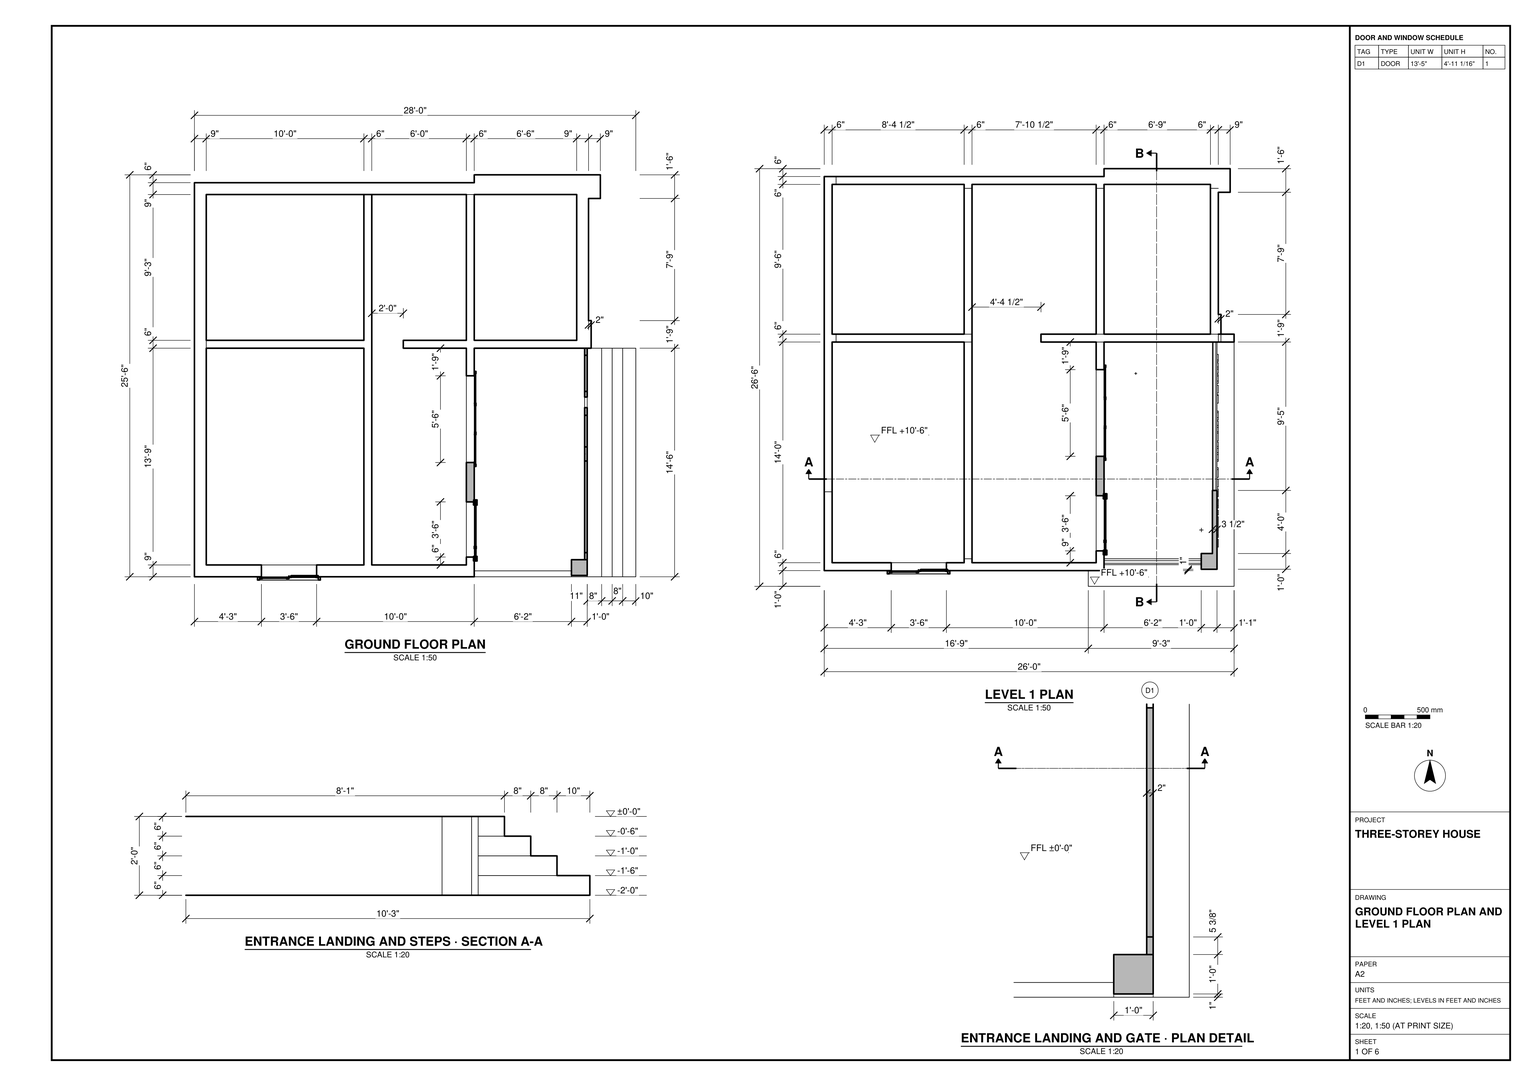
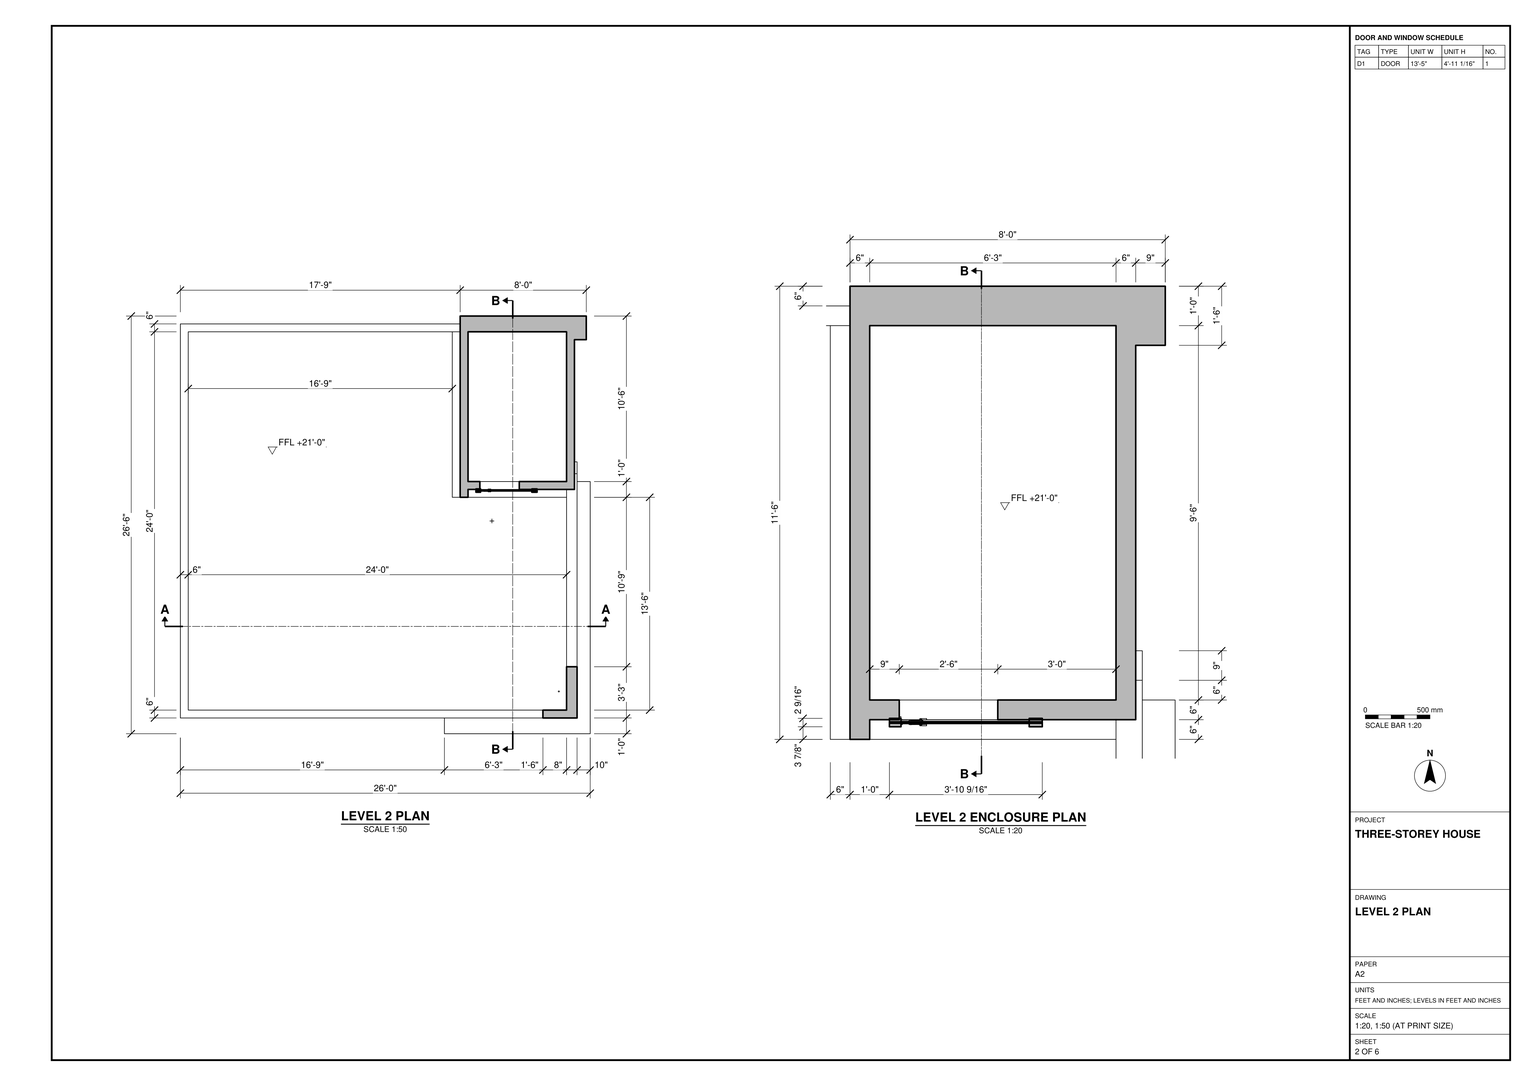
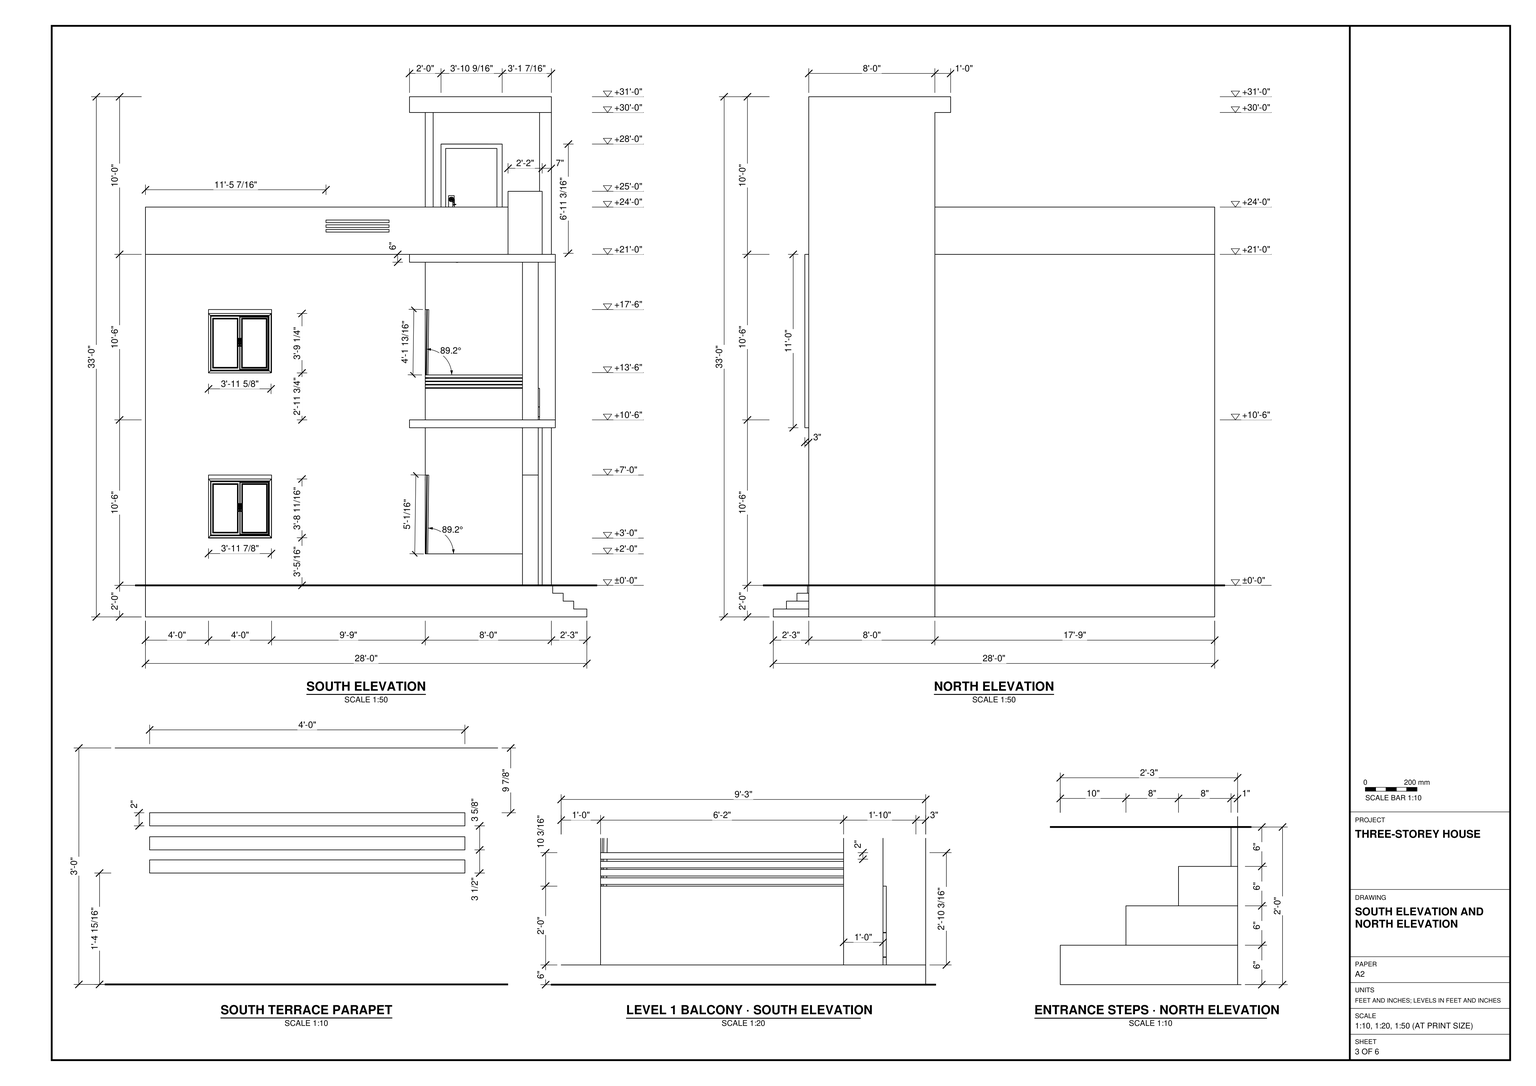
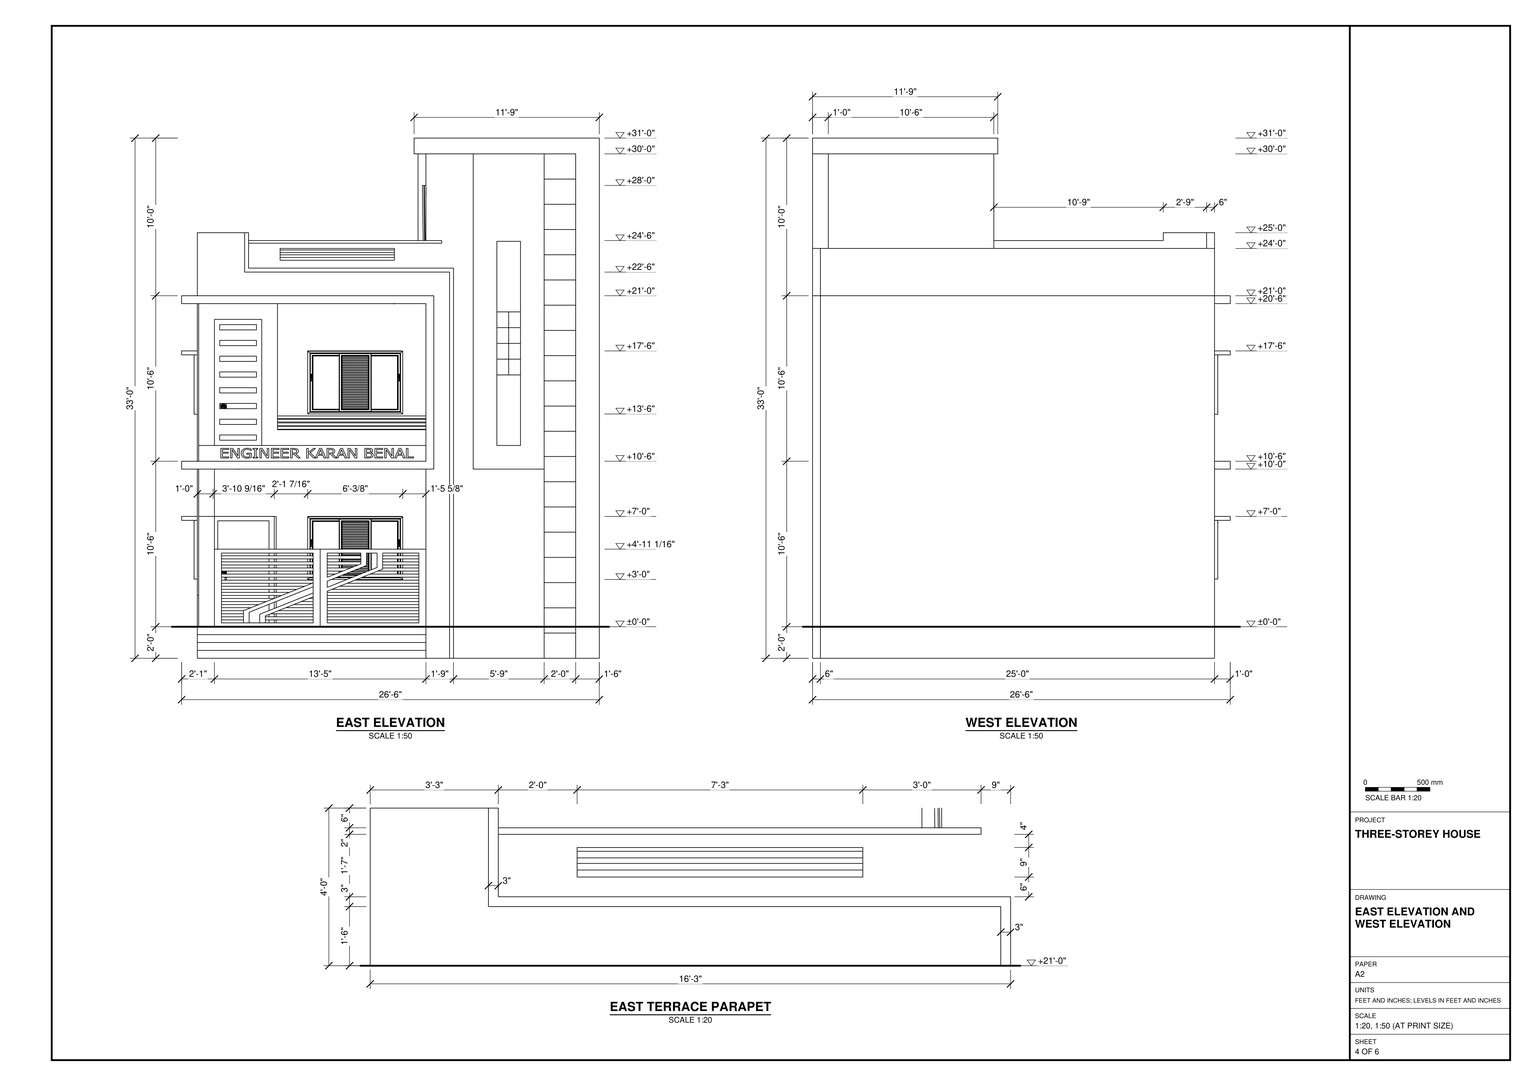
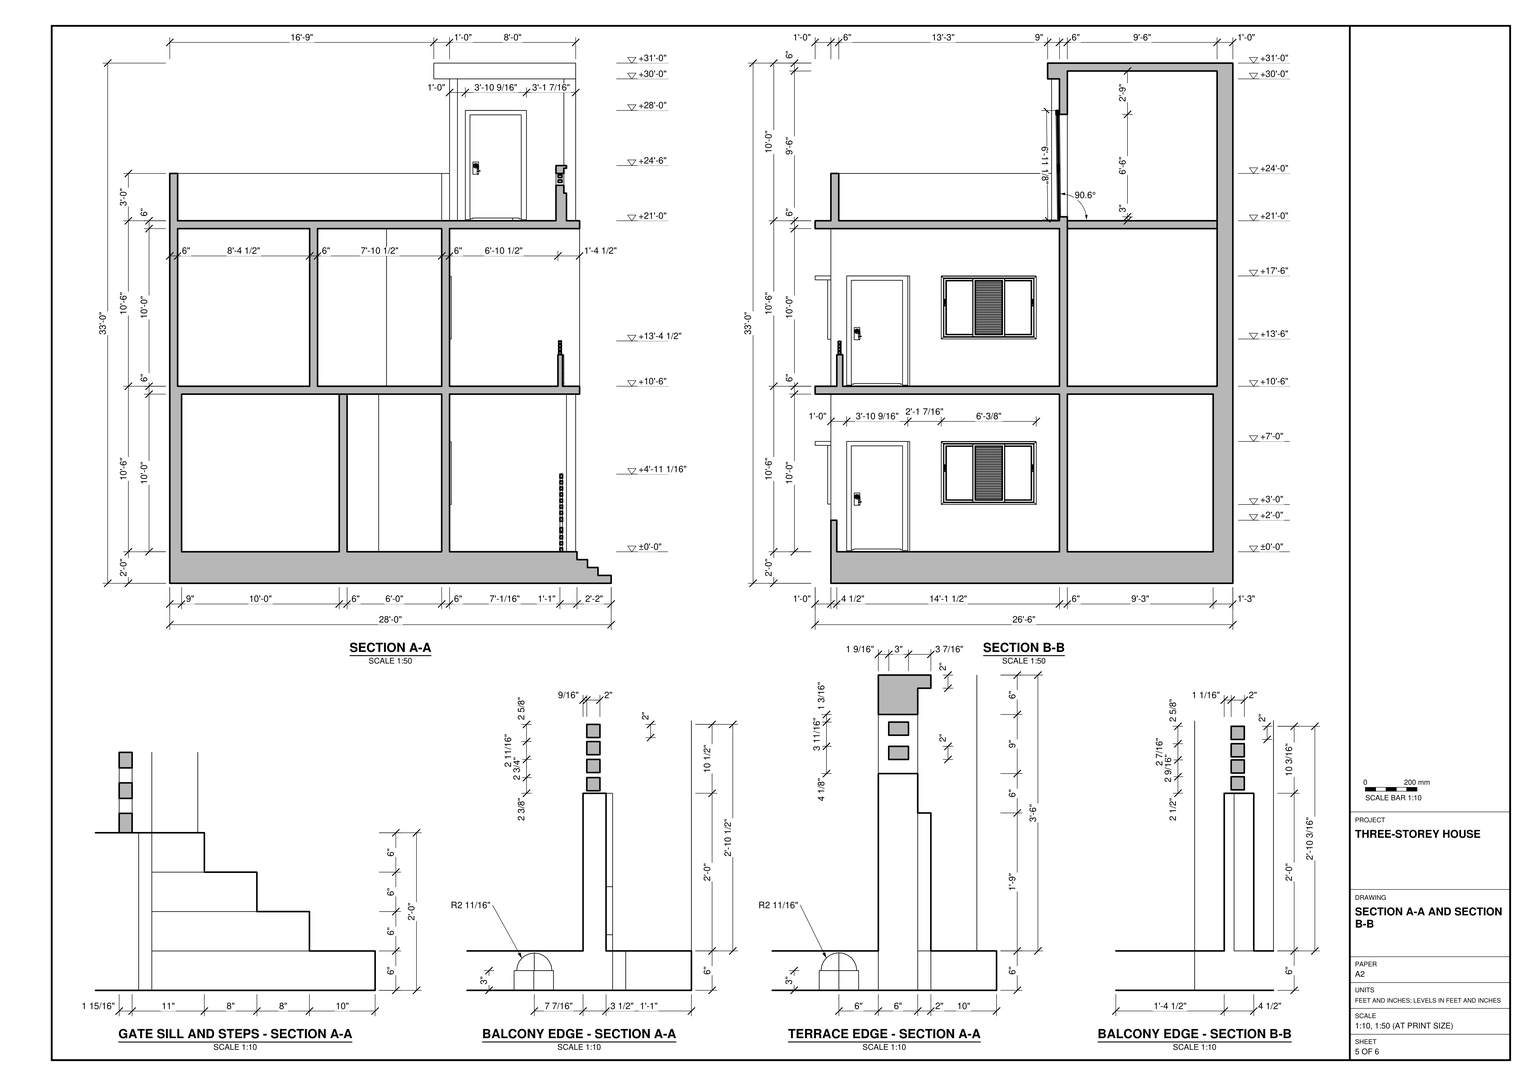
Build the house in SketchUp from task_files/diagram_01.pdf. Work in feet and inches. The overall extents are 28'-0" east to west, 26'-6" north to south and 33'-0" vertically. Set the ground floor at ±0'-0", level 1 at +10'-6" and level 2 at +21'-0". The overall height runs from the base of the entrance steps at -2'-0" to the top of the enclosure roof at +31'-0".

Lay out the lower floors from their respective plans. Follow the wall thicknesses, including the 9" ground-floor perimeter walls and 6" partitions where indicated. Keep the interior openings in their drawn positions rather than copying the ground-floor layout to level 1. Model the entrance landing, steps and gate on the east side, with the projecting balcony slab and horizontal railing above. Align the two south-facing window units as shown in elevation. At level 2, leave the terrace open around the northeast enclosure. Include the terrace parapet, its horizontal detail on the south face, and the enclosure's terrace-facing doorway and projecting flat roof.

Keep walls, slabs, roof elements and any furniture or joinery pieces in separate groups or components, and use components for repeated parts. Decor and loose items, if shown, may be any suitable library components. Save one SketchUp model as output_files/three_storey_house_with_a_balcony_and_roof_terrace.skp.

# SketchUp Ruby script. Lengths in inches.
U = 1.inch
M = Sketchup.active_model
def pt(a) = Geom::Point3d.new(a.map { |v| v * U })
def face(e, loops, mat)
  f = e.add_face(loops[0].map { |a| pt(a) })
  loops[1..].each { |l| e.add_face(l.map { |a| pt(a) }).erase! }
  f.material = f.back_material = mat if mat
  f
end
# faces: each face lists its corners as indices into pts; further lists are holes
def faces(e, pts, list, mat = nil) = list.each { |f| face(e, (f[0].is_a?(Array) ? f : [f]).map { |l| l.map { |i| pts[i] } }, mat) }
# xy, xz, yz: faces in a plane at the given z, y or x. An outline is a flat list of corners, or four numbers for a rectangle; further outlines are holes
def ring(l) = l.size == 4 ? [[l[0], l[1]], [l[2], l[1]], [l[2], l[3]], [l[0], l[3]]] : l.each_slice(2).to_a
def flat(e, list, mat, &to3) = list.each { |f| face(e, (f[0].is_a?(Array) ? f : [f]).map { |l| ring(l).map { |u, v| to3.(u, v) } }, mat) }
def xy(e, z, list, mat = nil) = flat(e, list, mat) { |x, y| [x, y, z] }
def xz(e, y, list, mat = nil) = flat(e, list, mat) { |x, z| [x, y, z] }
def yz(e, x, list, mat = nil) = flat(e, list, mat) { |y, z| [x, y, z] }
def lines(e, pts, list) = list.each { |a, b| e.add_line(pt(pts[a]), pt(pts[b])) }
# prism: a flat outline (further loops are holes) pulled along v
def prism(e, loops, v, mat = nil)
  f = face(e, loops, mat); d = Geom::Vector3d.new(v.map { |x| x * U })
  f.pushpull(f.normal.samedirection?(d) ? d.length : -d.length)
end
def box(e, o, s, mat = nil) = prism(e, [[o, [o[0] + s[0], o[1], o[2]], [o[0] + s[0], o[1] + s[1], o[2]], [o[0], o[1] + s[1], o[2]]]], [0, 0, s[2]], mat)
def at(x, y, z, deg = 0) = Geom::Transformation.translation(pt([x, y, z])) * Geom::Transformation.rotation(ORIGIN, Z_AXIS, deg.degrees)
def axes(o, x, y, z) = Geom::Transformation.new([*x, 0, *y, 0, *z, 0, *pt(o).to_a, 1])
def part(name) = M.definitions.add(name)
# library, detail: a bought-in or finely detailed component or shape, given as its bounding box
def library(name, o, s) = part(name).tap { |d| box(d.entities, o, s) }
def detail(e, o, s) = box(e.add_group.entities, o, s)
def put(e, d, t, mat = nil) = e.add_instance(d, t).tap { |i| i.material = mat if mat }
def group(e, t, mat = nil) = e.add_group.tap { |g| g.transformation = t; g.material = mat if mat }.entities
root = M.entities
M.materials.add("C03_Honey_Glow").color = [255, 178, 101]
M.materials.add("Carpet_04_1K").color = [43, 65, 85]
M.materials.add("D05_Goldenrod_Hue").color = [255, 191, 0]
M.materials.add("[_0053_Ivory_]").color = [200, 200, 200]
c1 = library("porta+4",[0.2,-5.42,1.33],[46.55,4.72,83.21])
c2 = library("Modern+Gate+1",[0,0,0],[118.11,1.97,78.74])
c3 = library("ENGINEER KARAN B",[0.96,0,0],[146.72,9.87,1])
c4 = library("Sphere Light",[-2.72,-2.72,-2.72],[5.44,5.44,5.44])
c5 = library("Sphere Light\#1",[-3.15,-3.15,-3.15],[6.3,6.3,6.3])
c6 = library("Sphere Light\#2",[-2.75,-2.75,-2.75],[5.5,5.5,5.5])
c7 = library("Sphere Light\#3",[-2.83,-2.83,-2.83],[5.66,5.66,5.66])
c8 = library("Sphere Light\#4",[-3.12,-3.12,-3.12],[6.24,6.24,6.24])
c9 = library("Sphere Light\#5",[-2.55,-2.55,-2.55],[5.1,5.1,5.1])
c10 = library("Sphere Light\#6",[-2.68,-2.68,-2.68],[5.36,5.36,5.36])
c11 = library("Sphere Light\#7",[-2.9,-2.9,-2.9],[5.8,5.8,5.8])
c12 = library("mesh-166",[-1553.69,-2604.3125,-42.18],[1702.88,1401.6,88.28])
c13 = part("Group17")
put(c13.entities,c12,at(294.66,859.51,3.5))
c14 = library("mesh-160",[-91.39,-1008.79,-36.9],[2366.42,1739.16,65.81])
c15 = part("Group4")
g1 = group(c15.entities,at(-5.75,-6.15,0))
put(g1,c14,axes([0,0,0],[1,0,0],[0,0,1],[0,-1,0]))
put(root,c1,at(224.8,188.76,275.46))
put(root,c1,at(210.24,23.8,23.48,90))
put(root,c1,at(210.24,23.8,149.48,90))
put(root,c2,axes([299,25,24],[0,1.36313,0],[-1,0,0],[0,0,0.75]))
g2 = group(root,at(0,72,0),"[_0053_Ivory_]")
xy(g2,0,[[0,-60,0,240,213,240,213,246,309,246,309,228,300,228,300,135,302,135,302,114,336,114,336,-60]])
xy(g2,6,[[326,-60,336,114]])
xy(g2,12,[[318,-60,326,114]])
xy(g2,18,[[310,-60,318,114]])
xy(g2,24,[[287,-60,299,-59],[299,-60,310,114],[213,-55.5,287,-55.5,287,-47,299,-47,299,114,213,114],[9,-51,129,114],[135,-51,207,-51,207,114,159,114,159,120,207,120,207,231,135,231],
  [9,120,129,231],[213,120,291,231]])
xy(g2,27,[[207,-45,213,-3]])
xy(g2,48,[[213,-60,287,-55.5]])
xy(g2,63,[[51,-60,93,-51],[207,27,213,93]])
xy(g2,105,[[48,-72,48,-60,51,-60,51,-51,93,-51,93,-60,96,-60,96,-72],[207,-45,213,-3],[207,27,213,93]])
xy(g2,108,[[48,-72,96,-60],[287,-59,299,-47]])
xy(g2,144,[[[201,-72,201,-60,213,-60,213,114,302,114,302,120,312,120,312,-72],[287,-59,299,-47],[237,87,237.78,87.1,238.5,87.4,239.12,87.88,239.6,88.5,239.9,89.22,240,90,239.9,90.78,239.6,91.5,239.12,92.12,238.5,92.6,237.78,92.9,237,93,236.22,92.9,235.5,92.6,234.88,92.12,234.4,91.5,234.1,90.78,234,90,234.1,89.22,234.4,88.5,234.88,87.88,235.5,87.4,236.22,87.1],[288,87,288.78,87.1,289.5,87.4,290.12,87.88,290.6,88.5,290.9,89.22,291,90,290.9,90.78,290.6,91.5,290.12,92.12,289.5,92.6,288.78,92.9,288,93,287.22,92.9,286.5,92.6,285.88,92.12,285.4,91.5,285.1,90.78,285,90,285.1,89.22,285.4,88.5,285.88,87.88,286.5,87.4,287.22,87.1],[237,-31.89,237.78,-31.79,238.5,-31.49,239.12,-31.01,239.6,-30.39,239.9,-29.66,240,-28.89,239.9,-28.11,239.6,-27.39,239.12,-26.77,238.5,-26.29,237.78,-25.99,237,-25.89,236.22,-25.99,235.5,-26.29,234.88,-26.77,234.4,-27.39,234.1,-28.11,234,-28.89,234.1,-29.66,234.4,-30.39,234.88,-31.01,235.5,-31.49,236.22,-31.79],[287.25,-31.88,288,-31.71,288.01,-31.71,288.71,-31.35,289.29,-30.83,289.71,-30.17,289.95,-29.42,289.99,-28.64,289.82,-27.875,289.47,-27.18,288.94,-26.6,288.28,-26.18,288,-26.08,287.54,-25.9375,286.75,-25.9,285.99,-26.0625,285.29,-26.42,284.71,-26.95,284.29,-27.61,284.05,-28.35,284.02,-28.89,284.01,-29.13,284.18,-29.9,284.53,-30.6,285.06,-31.18,285.72,-31.6,286.46,-31.84]],[287,-59,287,-48,288,-48,288,-47,299,-47,299,-59],[129,-51,135,-51,135,120,9,120,9,114,129,114],[9,-51,129,114],[135,-51,207,114],
  [287,-48,288,-47],[135,114,159,120],[9,120,129,231],[129,120,135,231],[135,120,207,231],
  [207,120,213,231],[213,120,291,231]])
xy(g2,147,[[237,-31.89,236.22,-31.79,235.5,-31.49,234.88,-31.01,234.4,-30.39,234.1,-29.66,234,-28.89,234.1,-28.11,234.4,-27.39,234.88,-26.77,235.5,-26.29,236.22,-25.99,237,-25.89,237.78,-25.99,238.5,-26.29,239.12,-26.77,239.6,-27.39,239.9,-28.11,240,-28.89,239.9,-29.66,239.6,-30.39,239.12,-31.01,238.5,-31.49,237.78,-31.79],[287.25,-31.88,286.46,-31.84,285.72,-31.6,285.06,-31.18,284.53,-30.6,284.18,-29.9,284.01,-29.13,284.02,-28.89,284.05,-28.35,284.29,-27.61,284.71,-26.95,285.29,-26.42,285.99,-26.0625,286.75,-25.9,287.54,-25.9375,288,-26.08,288.28,-26.18,288.94,-26.6,289.47,-27.18,289.82,-27.875,289.99,-28.64,289.95,-29.42,289.71,-30.17,289.29,-30.83,288.71,-31.35,288.01,-31.71,288,-31.71],[237,87,236.22,87.1,235.5,87.4,234.88,87.88,234.4,88.5,234.1,89.22,234,90,234.1,90.78,234.4,91.5,234.88,92.12,235.5,92.6,236.22,92.9,237,93,237.78,92.9,238.5,92.6,239.12,92.12,239.6,91.5,239.9,90.78,240,90,239.9,89.22,239.6,88.5,239.12,87.88,238.5,87.4,237.78,87.1],[288,87,287.22,87.1,286.5,87.4,285.88,87.88,285.4,88.5,285.1,89.22,285,90,285.1,90.78,285.4,91.5,285.88,92.12,286.5,92.6,287.22,92.9,288,93,288.78,92.9,289.5,92.6,290.12,92.12,290.6,91.5,290.9,90.78,291,90,290.9,89.22,290.6,88.5,290.12,87.88,289.5,87.4,288.78,87.1]])
xy(g2,150,[[201,-72,312,-72,312,114,299,114,299,-59,287,-59,287,-55.5,213,-55.5,213,-60,201,-60],[287,-59,299,-47],[6,-54,106.5,114],[112.5,-54,207,-54,207,114,165,114,165,120,207,120,207,234,112.5,234],[213,-51,287,-51,287,-47,295.5,-47,295.5,114,213,114],
  [6,120,106.5,234],[213,120,294,234]])
xy(g2,153,[[207,-45,213,-3]])
xy(g2,166,[[295.5,-43,299,-15]])
xy(g2,170,[[295.5,-43,299,-15]])
xy(g2,174,[[213,-55.5,287,-51],[295.5,1,299,114]])
xy(g2,174.39,[[296.07,1,298.07,114]])
xy(g2,174.52,[[213,-54.44,287,-52.44]])
xy(g2,176.39,[[296.07,1,298.07,114]])
xy(g2,176.52,[[213,-54.44,287,-52.44]])
xy(g2,177.08,[[213,-54.44,287,-52.44]])
xy(g2,177.16,[[296.07,1,298.07,114]])
xy(g2,178,[[295.5,-43,299,-15]])
xy(g2,179.08,[[213,-54.44,287,-52.44]])
xy(g2,179.16,[[296.07,1,298.07,114]])
xy(g2,179.55,[[213,-54.44,287,-52.44]])
xy(g2,179.875,[[296.07,1,298.07,114]])
xy(g2,181.55,[[213,-54.44,287,-52.44]])
xy(g2,181.875,[[296.07,1,298.07,114]])
xy(g2,182,[[295.5,-43,299,-15]])
xy(g2,182.2,[[213,-54.44,287,-52.44]])
xy(g2,182.49,[[296.07,1,298.07,114]])
xy(g2,184.2,[[213,-54.44,287,-52.44]])
xy(g2,184.49,[[296.07,1,298.07,114]])
xy(g2,189,[[51,-60,93,-54],[207,27,213,93]])
xy(g2,190,[[295.5,-43,299,-15]])
xy(g2,194,[[295.5,-43,299,-15]])
xy(g2,202,[[295.5,-43,299,-15]])
xy(g2,206,[[295.5,-43,299,-15]])
xy(g2,214,[[295.5,-43,299,-15]])
xy(g2,218,[[295.5,-43,299,-15]])
xy(g2,226,[[295.5,-43,299,-15]])
xy(g2,230,[[295.5,-43,299,-15]])
xy(g2,231,[[48,-72,48,-60,51,-60,51,-54,93,-54,93,-60,96,-60,96,-72],[207,-45,213,-3],[207,27,213,93]])
xy(g2,234,[[48,-72,96,-60]])
xy(g2,238,[[295.5,-43,299,-15]])
xy(g2,242,[[295.5,-43,299,-15]])
xy(g2,250,[[295.5,-43,299,-15]])
xy(g2,254,[[295.5,-43,299,-15]])
xy(g2,270,[[[201,-72,201,-60,213,-60,213,114,312,114,312,-72],[287,-59,299,-59,299,1,295.5,1,295.5,-47,287,-47],[237,-42.92,237.78,-42.82,238.5,-42.52,239.12,-42.04,239.6,-41.42,239.9,-40.7,240,-39.92,239.9,-39.14,239.6,-38.42,239.12,-37.8,238.5,-37.32,237.78,-37.02,237,-36.92,236.22,-37.02,235.5,-37.32,234.88,-37.8,234.4,-38.42,234.1,-39.14,234,-39.92,234.1,-40.7,234.4,-41.42,234.88,-42.04,235.5,-42.52,236.22,-42.82],[237,87,237.78,87.1,238.5,87.4,239.12,87.88,239.6,88.5,239.9,89.22,240,90,239.9,90.78,239.6,91.5,239.12,92.12,238.5,92.6,237.78,92.9,237,93,236.22,92.9,235.5,92.6,234.88,92.12,234.4,91.5,234.1,90.78,234,90,234.1,89.22,234.4,88.5,234.88,87.88,235.5,87.4,236.22,87.1],[288,87,288.78,87.1,289.5,87.4,290.12,87.88,290.6,88.5,290.9,89.22,291,90,290.9,90.78,290.6,91.5,290.12,92.12,289.5,92.6,288.78,92.9,288,93,287.22,92.9,286.5,92.6,285.88,92.12,285.4,91.5,285.1,90.78,285,90,285.1,89.22,285.4,88.5,285.88,87.88,286.5,87.4,287.22,87.1],[288,-42.92,288.78,-42.82,289.5,-42.52,290.12,-42.04,290.6,-41.42,290.9,-40.7,291,-39.92,290.9,-39.14,290.6,-38.42,290.12,-37.8,289.5,-37.32,288.78,-37.02,288,-36.92,287.22,-37.02,286.5,-37.32,285.88,-37.8,285.4,-38.42,285.1,-39.14,285,-39.92,285.1,-40.7,285.4,-41.42,285.88,-42.04,286.5,-42.52,287.22,-42.82]],[287,-59,287,-48,288,-48,288,-47,295.5,-47,295.5,1,299,1,299,-59],[6,-54,106.5,114],[112.5,-54,165,234],[165,-54,207,114],
  [287,-48,288,-47],[6,114,106.5,120],[165,114,207,120],[6,120,106.5,234],[165,120,207,234],
  [213,120,294,234]])
xy(g2,273,[[237,-42.92,236.22,-42.82,235.5,-42.52,234.88,-42.04,234.4,-41.42,234.1,-40.7,234,-39.92,234.1,-39.14,234.4,-38.42,234.88,-37.8,235.5,-37.32,236.22,-37.02,237,-36.92,237.78,-37.02,238.5,-37.32,239.12,-37.8,239.6,-38.42,239.9,-39.14,240,-39.92,239.9,-40.7,239.6,-41.42,239.12,-42.04,238.5,-42.52,237.78,-42.82],[288,-42.92,287.22,-42.82,286.5,-42.52,285.88,-42.04,285.4,-41.42,285.1,-40.7,285,-39.92,285.1,-39.14,285.4,-38.42,285.88,-37.8,286.5,-37.32,287.22,-37.02,288,-36.92,288.78,-37.02,289.5,-37.32,290.12,-37.8,290.6,-38.42,290.9,-39.14,291,-39.92,290.9,-40.7,290.6,-41.42,290.12,-42.04,289.5,-42.52,288.78,-42.82],[237,87,236.22,87.1,235.5,87.4,234.88,87.88,234.4,88.5,234.1,89.22,234,90,234.1,90.78,234.4,91.5,234.88,92.12,235.5,92.6,236.22,92.9,237,93,237.78,92.9,238.5,92.6,239.12,92.12,239.6,91.5,239.9,90.78,240,90,239.9,89.22,239.6,88.5,239.12,87.88,238.5,87.4,237.78,87.1],[288,87,287.22,87.1,286.5,87.4,285.88,87.88,285.4,88.5,285.1,89.22,285,90,285.1,90.78,285.4,91.5,285.88,92.12,286.5,92.6,287.22,92.9,288,93,288.78,92.9,289.5,92.6,290.12,92.12,290.6,91.5,290.9,90.78,291,90,290.9,89.22,290.6,88.5,290.12,87.88,289.5,87.4,288.78,87.1]])
xy(g2,276,[[201,-72,312,-72,312,120,302,120,302,-60,201,-60],[6,-54,294,-54,294,108,207,108,207,234,6,234],[207,108,213,234],[219,108,294,114],[213,120,219,234],
  [219,120,294,234]])
xy(g2,276,[[300,114,302,120]],"Carpet_04_1K")
xy(g2,279,[[228,114,258,120]])
xy(g2,292.96,[[137.43,-60,185.43,-54]])
xy(g2,294.96,[[137.43,-60,185.43,-54]])
xy(g2,296.49,[[137.43,-60,185.43,-54]])
xy(g2,297,[[300,-21,302,135]])
xy(g2,298.49,[[137.43,-60,185.43,-54]])
xy(g2,300.14,[[137.43,-60,185.43,-54]])
xy(g2,302.14,[[137.43,-60,185.43,-54]])
xy(g2,303,[[294,3,300,90]])
xy(g2,305.15,[[295.59,3,298.59,90]])
xy(g2,307.15,[[295.59,3,298.59,90]])
xy(g2,308.84,[[295.59,3,298.59,90]])
xy(g2,310.84,[[295.59,3,298.59,90]])
xy(g2,312,[[0,-60,276,-60,276,-54,6,-54,6,234,213,234,213,240,0,240],[294,3,300,90]])
xy(g2,316,[[300,-21,302,114],[300,114,302,126]])
xy(g2,318,[[294,-21,302,-21,302,126,300,126,300,114,294,114]])
xy(g2,324,[[276,-60,302,-60,302,-21,294,-21,294,-54,276,-54]])
xy(g2,357,[[228,114,258,120]])
xy(g2,384,[[201,105,201,114,213,114,213,108,219,108,219,114,300,114,300,228,309,228,309,105],[201,114,213,234],[201,234,213,246]])
xy(g2,390,[[219,120,294,234]])
xy(g2,396,[[201,105,309,246]])
xz(g2,-72,[[48,105,96,108],[201,144,312,150],[48,231,96,234],[201,270,312,276]])
xz(g2,-60,[[[0,0,336,0,336,6,326,6,326,12,318,12,318,18,310,18,310,24,287,24,287,48,213,48,213,144,201,144,201,150,213,150,213,270,201,270,201,276,0,276],[48,186,96,234],[48,60,96,108]],[48,60,96,60,96,105,93,105,93,63,51,63,51,105,48,105],[48,186,96,186,96,231,93,231,93,189,51,189,51,231,48,231],[[0,276,276,312],[137.43,300.14,185.43,302.14],[137.43,296.49,185.43,298.49],[137.43,292.96,185.43,294.96]]])
xz(g2,-60,[[276,276,302,324]],"Carpet_04_1K")
xz(g2,-59,[[287,108,299,144],[287,144,299,150],[287,150,299,270]])
xz(g2,-59,[[287,24,299,108]],"Carpet_04_1K")
xz(g2,-55.5,[[213,24,287,48],[213,150,287,174]])
xz(g2,-54.44,[[213,174.52,287,176.52],[213,177.08,287,179.08],[213,179.55,287,181.55],[213,182.2,287,184.2]])
xz(g2,-54,[[[6,150,106.5,270],[51,189,93,231]],[112.5,150,207,270],[[6,276,6,312,276,312,276,324,294,324,294,276],[137.43,292.96,185.43,294.96],[137.43,296.49,185.43,298.49],[137.43,300.14,185.43,302.14]]])
xz(g2,-52.44,[[213,174.52,287,176.52],[213,177.08,287,179.08],[213,179.55,287,181.55],[213,182.2,287,184.2]])
xz(g2,-51,[[[9,24,129,144],[51,63,93,105]],[135,24,207,144],[213,150,287,174]])
xz(g2,-47,[[287,108,299,144],[287,144,299,150],[287,150,295.5,270]])
xz(g2,-47,[[287,24,299,108]],"Carpet_04_1K")
xz(g2,-45,[[207,27,213,105],[207,153,213,231]])
xz(g2,-43,[[295.5,166,299,170],[295.5,178,299,182],[295.5,190,299,194],[295.5,202,299,206],[295.5,214,299,218],
  [295.5,226,299,230],[295.5,238,299,242],[295.5,250,299,254]])
xz(g2,-31.71,[[288,144,288.01,147]])
xz(g2,-21,[[300,297,302,316],[294,318,302,324]])
xz(g2,-15,[[295.5,166,299,170],[295.5,178,299,182],[295.5,190,299,194],[295.5,202,299,206],[295.5,214,299,218],
  [295.5,226,299,230],[295.5,238,299,242],[295.5,250,299,254]])
xz(g2,-3,[[207,27,213,105],[207,153,213,231]])
xz(g2,1,[[[295.5,174,299,270],[296.07,174.39,298.07,176.39],[296.07,177.16,298.07,179.16],[296.07,179.875,298.07,181.875],[296.07,182.49,298.07,184.49]]])
xz(g2,3,[[[294,303,300,312],[295.59,308.84,298.59,310.84],[295.59,305.15,298.59,307.15]]])
xz(g2,27,[[207,63,213,105],[207,189,213,231]])
xz(g2,90,[[[294,303,300,312],[295.59,308.84,298.59,310.84],[295.59,305.15,298.59,307.15]]])
xz(g2,93,[[207,63,213,105],[207,189,213,231]])
xz(g2,105,[[201,384,309,396]])
xz(g2,108,[[213,276,219,384]])
xz(g2,114,[[302,0,336,6],[302,6,326,12],[302,12,318,18],[302,18,310,24],[9,24,129,144],
  [159,24,207,144],[213,24,302,144],[6,150,106.5,270],[165,150,207,270],[[213,150,295.5,150,295.5,174,300,174,300,150,312,150,312,270,213,270],[296.07,182.49,298.07,184.49],[296.07,179.875,298.07,181.875],[296.07,177.16,298.07,179.16],[296.07,174.39,298.07,176.39]],
  [299,150,300,174],[219,276,225,276,225,360,261,360,261,276,294,276,294,318,300,318,300,384,219,384],[[225,276,261,360],[228,279,258,357]]])
xz(g2,120,[[9,24,129,144],[159,24,207,144],[213,24,291,144],[302,144,312,276],[6,150,106.5,270],
  [165,150,207,270],[213,150,294,270],[213,270,294,276],[[219,276,294,390],[228,279,258,357]]])
xz(g2,120,[[300,150,302,276]],"Carpet_04_1K")
xz(g2,126,[[300,316,302,318]])
xz(g2,135,[[300,0,302,297]])
xz(g2,228,[[300,0,309,384]])
xz(g2,231,[[9,24,129,144],[129,24,135,144],[135,24,207,144],[213,24,291,144]])
xz(g2,234,[[6,150,106.5,270],[112.5,150,207,270],[213,150,294,270],[213,270,294,276],[6,276,207,312],
  [207,276,213,312],[219,276,294,390]])
xz(g2,240,[[0,0,213,276],[0,276,213,312]])
xz(g2,246,[[213,0,213,384,201,384,201,396,309,396,309,0]])
yz(g2,0,[[-60,0,240,276],[-60,276,240,312]])
yz(g2,6,[[-54,150,114,270],[120,150,234,270],[-54,276,234,312]])
yz(g2,9,[[-51,24,114,144],[120,24,231,144]])
yz(g2,48,[[-72,105,-60,108],[-72,231,-60,234]])
yz(g2,51,[[-60,63,-51,105],[-60,189,-54,231]])
yz(g2,93,[[-60,63,-51,105],[-60,189,-54,231]])
yz(g2,96,[[-72,105,-60,108],[-72,231,-60,234]])
yz(g2,106.5,[[-54,150,114,270],[120,150,234,270]])
yz(g2,112.5,[[-54,150,234,270]])
yz(g2,129,[[-51,24,114,144],[120,24,231,144]])
yz(g2,135,[[-51,24,120,144],[120,24,231,144]])
yz(g2,137.43,[[-60,292.96,-54,294.96],[-60,296.49,-54,298.49],[-60,300.14,-54,302.14]])
yz(g2,159,[[114,24,120,144]])
yz(g2,165,[[114,150,120,270]])
yz(g2,185.43,[[-60,292.96,-54,294.96],[-60,296.49,-54,298.49],[-60,300.14,-54,302.14]])
yz(g2,201,[[-72,144,-60,150],[-72,270,-60,276],[105,384,246,396]])
yz(g2,207,[[[-51,24,114,144],[-45,27,-3,105],[27,63,93,105]],[120,24,231,144],[[-54,150,114,270],[-45,153,-3,231],[27,189,93,231]],[120,150,234,270]])
yz(g2,213,[[240,0,246,276],[[-55.5,24,-48,24,-48,108,0,108,0,24,114,24,114,144,-60,144,-60,48,-55.5,48],[24,60,96,108]],[[-48,24,0,108],[-45,27,-3,105]],[120,24,231,144],[[24,60,96,108],[27,63,93,105]],
  [[-60,150,-55.5,150,-55.5,174,-51,174,-51,150,-48,150,-48,234,0,234,0,150,114,150,114,270,-60,270],[24,186,96,234],[-54.44,174.52,-52.44,176.52],[-54.44,177.08,-52.44,179.08],[-54.44,179.55,-52.44,181.55],[-54.44,182.2,-52.44,184.2]],[[-48,150,0,234],[-45,153,-3,231]],[120,150,234,270],[-54.44,174.52,-52.44,176.52],[-54.44,177.08,-52.44,179.08],
  [-54.44,179.55,-52.44,181.55],[-54.44,182.2,-52.44,184.2],[[24,186,96,234],[27,189,93,231]],[114,270,120,276],[108,276,234,384],
  [240,276,246,312],[234,312,246,384]])
yz(g2,219,[[108,276,114,384],[120,276,234,390]])
yz(g2,228,[[114,279,120,357]])
yz(g2,258,[[114,279,120,357]])
yz(g2,276,[[-60,312,-54,324]])
yz(g2,287,[[-60,24,-59,48],[-59,24,-55.5,48],[-59,108,-47,144],[-59,144,-47,150],[[-59,150,-59,270,-47,270,-47,150,-51,150,-51,174,-55.5,174,-55.5,150],[-54.44,182.2,-52.44,184.2],[-54.44,179.55,-52.44,181.55],[-54.44,177.08,-52.44,179.08],[-54.44,174.52,-52.44,176.52]]])
yz(g2,287,[[-55.5,24,-55.5,48,-59,48,-59,108,-47,108,-47,24]],"Carpet_04_1K")
yz(g2,291,[[120,24,231,144]])
yz(g2,294,[[120,150,234,270],[120,270,234,276],[[-54,276,-54,324,-21,324,-21,318,108,318,108,276],[3,303,90,312]],[108,276,114,318],[120,276,234,390]])
yz(g2,295.5,[[[-47,150,114,174],[-43,166,-15,170]],[[-47,174,1,270],[-43,178,-15,182],[-43,190,-15,194],[-43,202,-15,206],[-43,214,-15,218],[-43,226,-15,230],[-43,250,-15,254],[-43,238,-15,242]]])
yz(g2,295.59,[[3,305.15,90,307.15],[3,308.84,90,310.84]])
yz(g2,296.07,[[1,174.39,114,176.39],[1,177.16,114,179.16],[1,179.875,114,181.875],[1,182.49,114,184.49]])
yz(g2,298.07,[[1,174.39,114,176.39],[1,177.16,114,179.16],[1,179.875,114,181.875],[1,182.49,114,184.49]])
yz(g2,298.59,[[3,305.15,90,307.15],[3,308.84,90,310.84]])
yz(g2,299,[[-59,108,-47,144],[-59,144,-47,150],[-59,162,-47,162,-47,258,-11,258,-11,162,114,162,114,174,1,174,1,270,-59,270],[[-47,162,-11,258],[-43,166,-15,170],[-43,190,-15,194],[-43,214,-15,218],[-43,238,-15,242],[-43,250,-15,254],[-43,226,-15,230],[-43,202,-15,206],[-43,178,-15,182]]])
yz(g2,299,[[-59,24,-47,108],[-59,150,114,162]],"Carpet_04_1K")
yz(g2,300,[[[135,0,204,0,204,144,150,144,150,384,114,384,114,318,126,318,126,316,-21,316,-21,297,135,297],[3,303,90,312]]])
yz(g2,300,[[168,162,186,215.71],[168,263.71,186,317.42]],"C03_Honey_Glow")
yz(g2,300,[[204,0,228,19.2],[204,19.2,228,38.4],[204,38.4,228,57.6],[204,57.6,228,76.8],[204,76.8,228,96],
  [204,96,228,115.2],[204,115.2,228,134.4],[204,134.4,228,153.6],[[150,144,204,384],[168,162,186,317.42]],[204,153.6,228,172.8],
  [204,172.8,228,192],[204,192,228,211.2],[204,211.2,228,230.4],[168,215.71,177,227.71],[177,215.71,186,227.71],
  [168,227.71,177,239.71],[177,227.71,186,239.71],[204,230.4,228,249.6],[168,239.71,177,251.71],[177,239.71,186,251.71],
  [204,249.6,228,268.8],[168,251.71,177,263.71],[177,251.71,186,263.71],[204,268.8,228,288],[204,288,228,307.2],
  [204,307.2,228,326.4],[204,326.4,228,345.6],[204,345.6,228,364.8],[204,364.8,228,384]],"Carpet_04_1K")
yz(g2,302,[[132,0,135,0,135,297,-21,297,-21,324,-24,324,-24,294,132,294],[-21,316,126,318]])
yz(g2,302,[[114,0,132,0,132,294,-24,294,-24,324,-60,324,-60,276,120,276,120,144,114,144]],"Carpet_04_1K")
yz(g2,309,[[228,0,246,0,246,396,105,396,105,384,228,384]])
yz(g2,310,[[-60,18,114,24]])
yz(g2,312,[[-72,144,120,144,120,276,-72,276,-72,270,114,270,114,150,-72,150]])
yz(g2,318,[[-60,12,114,18]])
yz(g2,326,[[-60,6,114,12]])
yz(g2,336,[[-60,0,114,6]])
p = [[237,-31.89,144],[236.22,-31.79,144],[236.22,-31.79,147],[237,-31.89,147],[237.78,-31.79,144],[237.78,-31.79,147],
  [287.25,-31.88,144],[286.46,-31.84,144],[286.46,-31.84,147],[287.25,-31.88,147],[288,-31.71,144],[288,-31.71,147],
  [235.5,-31.49,144],[235.5,-31.49,147],[238.5,-31.49,144],[238.5,-31.49,147],[285.72,-31.6,144],[285.72,-31.6,147],
  [288.71,-31.35,144],[288.01,-31.71,144],[288.01,-31.71,147],[288.71,-31.35,147],[285.06,-31.18,144],[285.06,-31.18,147],
  [234.88,-31.01,144],[234.88,-31.01,147],[239.12,-31.01,144],[239.12,-31.01,147],[289.29,-30.83,144],[289.29,-30.83,147],
  [284.53,-30.6,144],[284.53,-30.6,147],[234.4,-30.39,144],[234.4,-30.39,147],[239.6,-30.39,144],[239.6,-30.39,147],
  [289.71,-30.17,144],[289.71,-30.17,147],[284.18,-29.9,144],[284.18,-29.9,147],[234.1,-29.66,144],[234.1,-29.66,147],
  [239.9,-29.66,144],[239.9,-29.66,147],[289.95,-29.42,144],[289.95,-29.42,147],[284.01,-29.13,144],[284.01,-29.13,147],
  [234,-28.89,144],[234,-28.89,147],[240,-28.89,144],[240,-28.89,147],[289.99,-28.64,144],[289.99,-28.64,147],
  [284.02,-28.89,144],[284.02,-28.89,147],[234.1,-28.11,144],[234.1,-28.11,147],[239.9,-28.11,144],[239.9,-28.11,147],
  [284.05,-28.35,144],[284.05,-28.35,147],[289.82,-27.875,144],[289.82,-27.875,147],[284.29,-27.61,144],[284.29,-27.61,147],
  [234.4,-27.39,144],[234.4,-27.39,147],[239.6,-27.39,144],[239.6,-27.39,147],[289.47,-27.18,144],[289.47,-27.18,147],
  [284.71,-26.95,144],[284.71,-26.95,147],[234.88,-26.77,144],[234.88,-26.77,147],[239.12,-26.77,144],[239.12,-26.77,147],
  [288.94,-26.6,144],[288.94,-26.6,147],[285.29,-26.42,144],[285.29,-26.42,147],[235.5,-26.29,144],[235.5,-26.29,147],
  [238.5,-26.29,144],[238.5,-26.29,147],[288.28,-26.18,144],[288.28,-26.18,147],[285.99,-26.0625,144],[285.99,-26.0625,147],
  [236.22,-25.99,144],[236.22,-25.99,147],[237.78,-25.99,144],[237.78,-25.99,147],[288,-26.08,144],[288,-26.08,147],
  [286.75,-25.9,144],[286.75,-25.9,147],[287.54,-25.9375,144],[287.54,-25.9375,147],[237,-25.89,144],[237,-25.89,147],
  [237,87,144],[236.22,87.1,144],[236.22,87.1,147],[237,87,147],[237.78,87.1,144],[237.78,87.1,147],
  [288,87,144],[287.22,87.1,144],[287.22,87.1,147],[288,87,147],[288.78,87.1,144],[288.78,87.1,147],
  [235.5,87.4,144],[235.5,87.4,147],[238.5,87.4,144],[238.5,87.4,147],[286.5,87.4,144],[286.5,87.4,147],
  [289.5,87.4,144],[289.5,87.4,147],[234.88,87.88,144],[234.88,87.88,147],[239.12,87.88,144],[239.12,87.88,147],
  [285.88,87.88,144],[285.88,87.88,147],[290.12,87.88,144],[290.12,87.88,147],[234.4,88.5,144],[234.4,88.5,147],
  [239.6,88.5,144],[239.6,88.5,147],[285.4,88.5,144],[285.4,88.5,147],[290.6,88.5,144],[290.6,88.5,147],
  [234.1,89.22,144],[234.1,89.22,147],[239.9,89.22,144],[239.9,89.22,147],[285.1,89.22,144],[285.1,89.22,147],
  [290.9,89.22,144],[290.9,89.22,147],[234,90,144],[234,90,147],[240,90,144],[240,90,147],
  [285,90,144],[285,90,147],[291,90,144],[291,90,147],[234.1,90.78,144],[234.1,90.78,147],
  [239.9,90.78,144],[239.9,90.78,147],[285.1,90.78,144],[285.1,90.78,147],[290.9,90.78,144],[290.9,90.78,147],
  [234.4,91.5,144],[234.4,91.5,147],[239.6,91.5,144],[239.6,91.5,147],[285.4,91.5,144],[285.4,91.5,147],
  [290.6,91.5,144],[290.6,91.5,147],[234.88,92.12,144],[234.88,92.12,147],[239.12,92.12,144],[239.12,92.12,147],
  [285.88,92.12,144],[285.88,92.12,147],[290.12,92.12,144],[290.12,92.12,147],[235.5,92.6,144],[235.5,92.6,147],
  [238.5,92.6,144],[238.5,92.6,147],[286.5,92.6,144],[286.5,92.6,147],[289.5,92.6,144],[289.5,92.6,147],
  [236.22,92.9,144],[236.22,92.9,147],[237.78,92.9,144],[237.78,92.9,147],[287.22,92.9,144],[287.22,92.9,147],
  [288.78,92.9,144],[288.78,92.9,147],[237,93,144],[237,93,147],[288,93,144],[288,93,147],
  [237,-42.92,270],[236.22,-42.82,270],[236.22,-42.82,273],[237,-42.92,273],[237.78,-42.82,270],[237.78,-42.82,273],
  [288,-42.92,270],[287.22,-42.82,270],[287.22,-42.82,273],[288,-42.92,273],[288.78,-42.82,270],[288.78,-42.82,273],
  [235.5,-42.52,270],[235.5,-42.52,273],[238.5,-42.52,270],[238.5,-42.52,273],[286.5,-42.52,270],[286.5,-42.52,273],
  [289.5,-42.52,270],[289.5,-42.52,273],[234.88,-42.04,270],[234.88,-42.04,273],[239.12,-42.04,270],[239.12,-42.04,273],
  [285.88,-42.04,270],[285.88,-42.04,273],[290.12,-42.04,270],[290.12,-42.04,273],[234.4,-41.42,270],[234.4,-41.42,273],
  [239.6,-41.42,270],[239.6,-41.42,273],[285.4,-41.42,270],[285.4,-41.42,273],[290.6,-41.42,270],[290.6,-41.42,273],
  [234.1,-40.7,270],[234.1,-40.7,273],[239.9,-40.7,270],[239.9,-40.7,273],[285.1,-40.7,270],[285.1,-40.7,273],
  [290.9,-40.7,270],[290.9,-40.7,273],[234,-39.92,270],[234,-39.92,273],[240,-39.92,270],[240,-39.92,273],
  [285,-39.92,270],[285,-39.92,273],[291,-39.92,270],[291,-39.92,273],[234.1,-39.14,270],[234.1,-39.14,273],
  [239.9,-39.14,270],[239.9,-39.14,273],[285.1,-39.14,270],[285.1,-39.14,273],[290.9,-39.14,270],[290.9,-39.14,273],
  [234.4,-38.42,270],[234.4,-38.42,273],[239.6,-38.42,270],[239.6,-38.42,273],[285.4,-38.42,270],[285.4,-38.42,273],
  [290.6,-38.42,270],[290.6,-38.42,273],[234.88,-37.8,270],[234.88,-37.8,273],[239.12,-37.8,270],[239.12,-37.8,273],
  [285.88,-37.8,270],[285.88,-37.8,273],[290.12,-37.8,270],[290.12,-37.8,273],[235.5,-37.32,270],[235.5,-37.32,273],
  [238.5,-37.32,270],[238.5,-37.32,273],[286.5,-37.32,270],[286.5,-37.32,273],[289.5,-37.32,270],[289.5,-37.32,273],
  [236.22,-37.02,270],[236.22,-37.02,273],[237.78,-37.02,270],[237.78,-37.02,273],[287.22,-37.02,270],[287.22,-37.02,273],
  [288.78,-37.02,270],[288.78,-37.02,273],[237,-36.92,270],[237,-36.92,273],[288,-36.92,270],[288,-36.92,273],
  [237,87,270],[236.22,87.1,270],[236.22,87.1,273],[237,87,273],[237.78,87.1,270],[237.78,87.1,273],
  [288,87,270],[287.22,87.1,270],[287.22,87.1,273],[288,87,273],[288.78,87.1,270],[288.78,87.1,273],
  [235.5,87.4,270],[235.5,87.4,273],[238.5,87.4,270],[238.5,87.4,273],[286.5,87.4,270],[286.5,87.4,273],
  [289.5,87.4,270],[289.5,87.4,273],[234.88,87.88,270],[234.88,87.88,273],[239.12,87.88,270],[239.12,87.88,273],
  [285.88,87.88,270],[285.88,87.88,273],[290.12,87.88,270],[290.12,87.88,273],[234.4,88.5,270],[234.4,88.5,273],
  [239.6,88.5,270],[239.6,88.5,273],[285.4,88.5,270],[285.4,88.5,273],[290.6,88.5,270],[290.6,88.5,273],
  [234.1,89.22,270],[234.1,89.22,273],[239.9,89.22,270],[239.9,89.22,273],[285.1,89.22,270],[285.1,89.22,273],
  [290.9,89.22,270],[290.9,89.22,273],[234,90,270],[234,90,273],[240,90,270],[240,90,273],
  [285,90,270],[285,90,273],[291,90,270],[291,90,273],[234.1,90.78,270],[234.1,90.78,273],
  [239.9,90.78,270],[239.9,90.78,273],[285.1,90.78,270],[285.1,90.78,273],[290.9,90.78,270],[290.9,90.78,273],
  [234.4,91.5,270],[234.4,91.5,273],[239.6,91.5,270],[239.6,91.5,273],[285.4,91.5,270],[285.4,91.5,273],
  [290.6,91.5,270],[290.6,91.5,273],[234.88,92.12,270],[234.88,92.12,273],[239.12,92.12,270],[239.12,92.12,273],
  [285.88,92.12,270],[285.88,92.12,273],[290.12,92.12,270],[290.12,92.12,273],[235.5,92.6,270],[235.5,92.6,273],
  [238.5,92.6,270],[238.5,92.6,273],[286.5,92.6,270],[286.5,92.6,273],[289.5,92.6,270],[289.5,92.6,273],
  [236.22,92.9,270],[236.22,92.9,273],[237.78,92.9,270],[237.78,92.9,273],[287.22,92.9,270],[287.22,92.9,273],
  [288.78,92.9,270],[288.78,92.9,273],[237,93,270],[237,93,273],[288,93,270],[288,93,273],
  [9,9,0],[9,9,24],[291,9,0],[291,9,24],[291,231,0],[291,231,24],
  [9,231,0],[9,231,24],[213,231,24],[207,231,24],[0,0,144],[9,0,144],
  [9,231,144],[9,240,144],[9,120,24],[9,114,24],[291,120,144],[300,120,144],
  [291,231,144],[300,231,144],[6,234,270],[6,240,270],[213,114,144],[207,114,144],
  [6,-54,270],[6,-60,270],[106.5,-54,270],[106.5,-60,270],[207,-54,270],[207,-60,270],
  [165,-54,270],[165,-60,270],[300,114,270],[300,114,276],[300,114,150],[300,120,150],
  [299,-47,174],[295.5,-47,174],[285.1,-39.92,270]]
faces(g2,p,[[0,1,2,3],[4,0,3,5],[6,7,8,9],[10,6,9,11],[1,12,13,2],[14,4,5,15],[7,16,17,8],[18,19,20,21],
  [16,22,23,17],[12,24,25,13],[26,14,15,27],[28,18,21,29],[22,30,31,23],[24,32,33,25],[34,26,27,35],[36,28,29,37],
  [30,38,39,31],[32,40,41,33],[42,34,35,43],[44,36,37,45],[38,46,47,39],[40,48,49,41],[50,42,43,51],[52,44,45,53],
  [46,54,55,47],[48,56,57,49],[58,50,51,59],[54,60,61,55],[62,52,53,63],[60,64,65,61],[56,66,67,57],[68,58,59,69],
  [70,62,63,71],[64,72,73,65],[66,74,75,67],[76,68,69,77],[78,70,71,79],[72,80,81,73],[74,82,83,75],[84,76,77,85],
  [86,78,79,87],[80,88,89,81],[82,90,91,83],[92,84,85,93],[94,86,87,95],[88,96,97,89],[98,94,95,99],[90,100,101,91],
  [100,92,93,101],[96,98,99,97],[102,103,104,105],[106,102,105,107],[108,109,110,111],[112,108,111,113],[103,114,115,104],[116,106,107,117],
  [109,118,119,110],[120,112,113,121],[114,122,123,115],[124,116,117,125],[118,126,127,119],[128,120,121,129],[122,130,131,123],[132,124,125,133],
  [126,134,135,127],[136,128,129,137],[130,138,139,131],[140,132,133,141],[134,142,143,135],[144,136,137,145],[138,146,147,139],[148,140,141,149],
  [142,150,151,143],[152,144,145,153],[146,154,155,147],[156,148,149,157],[150,158,159,151],[160,152,153,161],[154,162,163,155],[164,156,157,165],
  [158,166,167,159],[168,160,161,169],[162,170,171,163],[172,164,165,173],[166,174,175,167],[176,168,169,177],[170,178,179,171],[180,172,173,181],
  [174,182,183,175],[184,176,177,185],[178,186,187,179],[188,180,181,189],[182,190,191,183],[192,184,185,193],[186,194,195,187],[194,188,189,195],
  [190,196,197,191],[196,192,193,197],[198,199,200,201],[202,198,201,203],[204,205,206,207],[208,204,207,209],[199,210,211,200],[212,202,203,213],
  [205,214,215,206],[216,208,209,217],[210,218,219,211],[220,212,213,221],[214,222,223,215],[224,216,217,225],[218,226,227,219],[228,220,221,229],
  [222,230,231,223],[232,224,225,233],[226,234,235,227],[236,228,229,237],[230,238,239,231],[240,232,233,241],[234,242,243,235],[244,236,237,245],
  [238,246,247,239],[248,240,241,249],[242,250,251,243],[252,244,245,253],[246,254,255,247],[256,248,249,257],[250,258,259,251],[260,252,253,261],
  [254,262,263,255],[264,256,257,265],[258,266,267,259],[268,260,261,269],[262,270,271,263],[272,264,265,273],[266,274,275,267],[276,268,269,277],
  [270,278,279,271],[280,272,273,281],[274,282,283,275],[284,276,277,285],[278,286,287,279],[288,280,281,289],[282,290,291,283],[290,284,285,291],
  [286,292,293,287],[292,288,289,293],[294,295,296,297],[298,294,297,299],[300,301,302,303],[304,300,303,305],[295,306,307,296],[308,298,299,309],
  [301,310,311,302],[312,304,305,313],[306,314,315,307],[316,308,309,317],[310,318,319,311],[320,312,313,321],[314,322,323,315],[324,316,317,325],
  [318,326,327,319],[328,320,321,329],[322,330,331,323],[332,324,325,333],[326,334,335,327],[336,328,329,337],[330,338,339,331],[340,332,333,341],
  [334,342,343,335],[344,336,337,345],[338,346,347,339],[348,340,341,349],[342,350,351,343],[352,344,345,353],[346,354,355,347],[356,348,349,357],
  [350,358,359,351],[360,352,353,361],[354,362,363,355],[364,356,357,365],[358,366,367,359],[368,360,361,369],[362,370,371,363],[372,364,365,373],
  [366,374,375,367],[376,368,369,377],[370,378,379,371],[380,372,373,381],[374,382,383,375],[384,376,377,385],[378,386,387,379],[386,380,381,387],
  [382,388,389,383],[388,384,385,389]])
lines(g2,p,[[390,391],[392,393],[394,395],[396,397],[398,399],[400,401],[402,403],[404,405],[406,407],[408,409],[410,411],[412,413],
  [414,415],[416,417],[418,419],[420,421],[422,423],[424,425],[426,427],[246,428]])
put(g2,c3,axes([299,-43.09,152.32],[0,1,0],[0,0,0.77],[1,0,0]),"D05_Goldenrod_Hue")
put(g2,c4,at(288,90,273))
put(g2,c5,at(237.17,89.98,273))
put(g2,c6,at(236.95,-40.05,273))
put(g2,c7,at(288.125,-39.8,273))
put(g2,c8,at(287.08,-29.09,147))
put(g2,c9,at(236.96,-29.06,147))
put(g2,c10,at(288.08,90,147))
put(g2,c11,at(237.17,90.0625,147))
put(root,c13,axes([83.39,11.36,115.93],[0.02811,0,0],[0,0,0.03189],[0,-0.03937,0]))
put(root,c13,axes([83.19,11.36,242.08],[0.02795,0,0],[0,0,0.03228],[0,-0.03937,0]))
put(root,c15,axes([213.64,98.97,87.69],[0,0.03058,0],[-0.0208,0,0],[0,0,0.02744]))
put(root,c15,axes([213.64,98.97,213.69],[0,0.03058,0],[-0.0208,0,0],[0,0,0.02744]))
